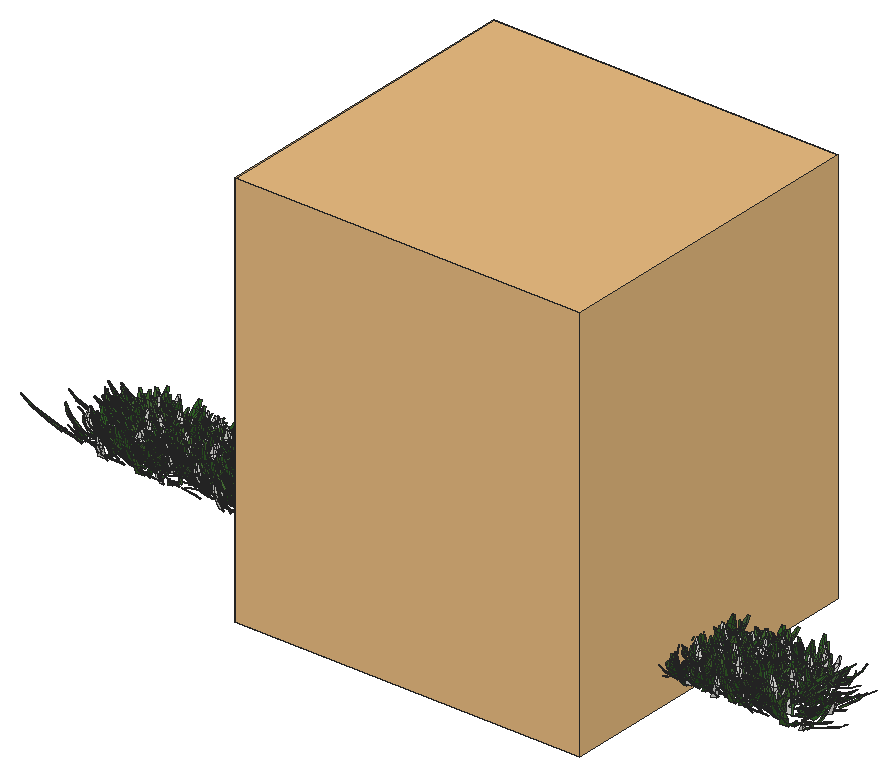
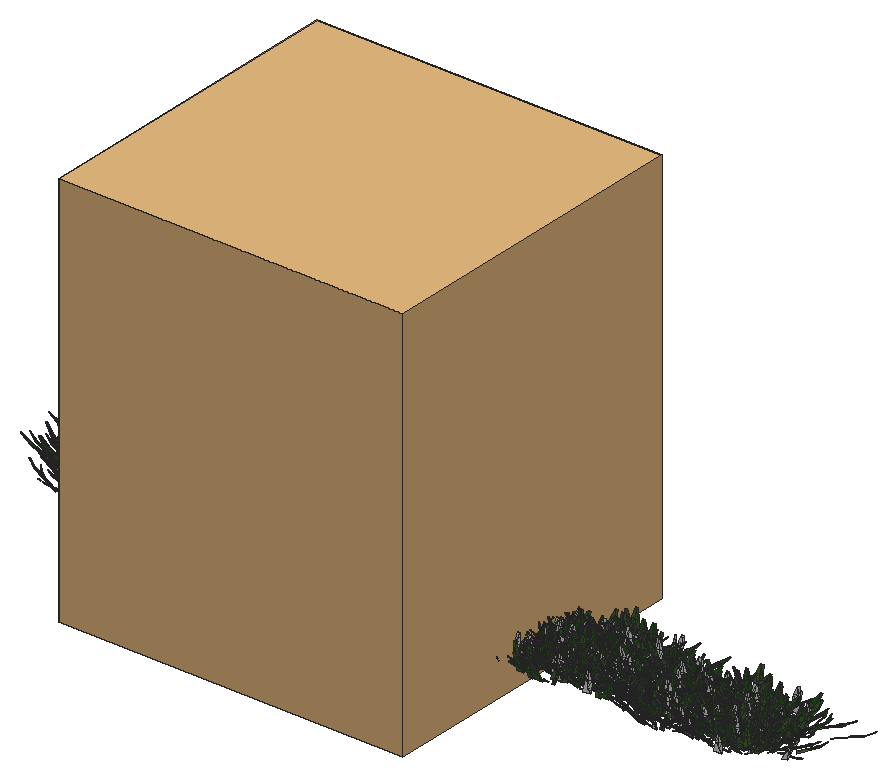
# SketchUp Ruby script. Lengths in inches.
U = 1.inch
M = Sketchup.active_model
def pt(a) = Geom::Point3d.new(a.map { |v| v * U })
def face(e, loops, mat)
  f = e.add_face(loops[0].map { |a| pt(a) })
  loops[1..].each { |l| e.add_face(l.map { |a| pt(a) }).erase! }
  f.material = f.back_material = mat if mat
  f
end
# faces: each face lists its corners as indices into pts; further lists are holes
def faces(e, pts, list, mat = nil) = list.each { |f| face(e, (f[0].is_a?(Array) ? f : [f]).map { |l| l.map { |i| pts[i] } }, mat) }
# xy, xz, yz: faces in a plane at the given z, y or x. An outline is a flat list of corners, or four numbers for a rectangle; further outlines are holes
def ring(l) = l.size == 4 ? [[l[0], l[1]], [l[2], l[1]], [l[2], l[3]], [l[0], l[3]]] : l.each_slice(2).to_a
def flat(e, list, mat, &to3) = list.each { |f| face(e, (f[0].is_a?(Array) ? f : [f]).map { |l| ring(l).map { |u, v| to3.(u, v) } }, mat) }
def xy(e, z, list, mat = nil) = flat(e, list, mat) { |x, y| [x, y, z] }
def xz(e, y, list, mat = nil) = flat(e, list, mat) { |x, z| [x, y, z] }
def yz(e, x, list, mat = nil) = flat(e, list, mat) { |y, z| [x, y, z] }
def lines(e, pts, list) = list.each { |a, b| e.add_line(pt(pts[a]), pt(pts[b])) }
# prism: a flat outline (further loops are holes) pulled along v
def prism(e, loops, v, mat = nil)
  f = face(e, loops, mat); d = Geom::Vector3d.new(v.map { |x| x * U })
  f.pushpull(f.normal.samedirection?(d) ? d.length : -d.length)
end
def box(e, o, s, mat = nil) = prism(e, [[o, [o[0] + s[0], o[1], o[2]], [o[0] + s[0], o[1] + s[1], o[2]], [o[0], o[1] + s[1], o[2]]]], [0, 0, s[2]], mat)
def at(x, y, z, deg = 0) = Geom::Transformation.translation(pt([x, y, z])) * Geom::Transformation.rotation(ORIGIN, Z_AXIS, deg.degrees)
def axes(o, x, y, z) = Geom::Transformation.new([*x, 0, *y, 0, *z, 0, *pt(o).to_a, 1])
def part(name) = M.definitions.add(name)
# library, detail: a bought-in or finely detailed component or shape, given as its bounding box
def library(name, o, s) = part(name).tap { |d| box(d.entities, o, s) }
def detail(e, o, s) = box(e.add_group.entities, o, s)
def put(e, d, t, mat = nil) = e.add_instance(d, t).tap { |i| i.material = mat if mat }
def group(e, t, mat = nil) = e.add_group.tap { |g| g.transformation = t; g.material = mat if mat }.entities
root = M.entities
M.materials.add("Material82").color = [68, 110, 58]
M.materials.add("Material83").color = [48, 90, 38]
M.materials.add("Material84").color = [68, 110, 48]
M.materials.add("Material85").color = [48, 90, 48]
M.materials.add("Material86").color = [58, 110, 58]
M.materials.add("Material87").color = [58, 90, 38]
M.materials.add("Material88").color = [68, 100, 58]
M.materials.add("Material89").color = [48, 100, 38]
c1 = part("grass00")
p = [[-0.6875,0.15,0],[-0.56,0.08,5.52],[-0.04,0.03,2.76],[0.48,-0.02,0],[0.35,-0.02,5.52],[-0.1,-0.14,5.52],
  [-0.12,0.65,8.37],[-0.42,0.65,8.37]]
faces(c1.entities,p,[[0,1,2,3],[3,2,4],[1,5,2],[5,4,2],[1,6,5],[4,5,6],[7,6,1]])
c2 = part("Group16\#1")
put(c2.entities,c1,axes([1.44,-0.61,-0.01],[0.05352,0.12609,0],[-0.10704,0.04543,0.07239],[0.06664,-0.02828,0.11628]),"Material85")
put(c2.entities,c1,axes([0.76,-0.15,-0.01],[0.04676,0.24062,0],[-0.23162,0.04501,0.06642],[0.0652,-0.01267,0.23595]),"Material82")
put(c2.entities,c1,axes([0.79,0.01,-0.01],[-0.00606,0.34651,0],[-0.34381,-0.00602,0.0432],[0.04319,0.00076,0.34386]))
put(c2.entities,c1,axes([1,0.23,-0.01],[-0.07192,0.31144,0],[-0.28722,-0.06632,0.1236],[0.12043,0.02781,0.29478]),"Material84")
put(c2.entities,c1,axes([1.66,0.77,-0.01],[-0.13828,0.29651,0],[-0.21551,-0.1005,0.22471],[0.20365,0.09498,0.23779]),"Material89")
put(c2.entities,c1,axes([0.6875,0.52,-0.01],[-0.18126,0.24051,0],[-0.22746,-0.17142,0.09788],[0.07817,0.05891,0.28481]),"Material84")
put(c2.entities,c1,axes([0.68,0.78,-0.01],[-0.215,0.18688,0],[-0.12385,-0.14248,0.21334],[0.13995,0.16101,0.18878]),"Material82")
put(c2.entities,c1,axes([0.56,1,-0.01],[-0.13756,0.07624,0],[-0.06159,-0.11112,0.0927],[0.04494,0.08108,0.12705]),"Material84")
put(c2.entities,c1,axes([0.2,0.64,-0.01],[-0.23729,0.07254,0],[-0.05711,-0.18681,0.153],[0.04473,0.14632,0.19535]),"Material89")
put(c2.entities,c1,axes([0.0625,0.72,-0.01],[-0.28874,0.02525,0],[-0.02179,-0.24916,0.14647],[0.01276,0.14591,0.25012]),"Material82")
put(c2.entities,c1,axes([-0.08,0.62,-0.01],[-0.34089,-0.04187,0],[0.03255,-0.26504,0.216],[-0.02633,0.21439,0.26703]),"Material89")
put(c2.entities,c1,axes([-0.34,0.98,-0.01],[-0.14314,-0.0493,0],[0.04397,-0.12769,0.06843],[-0.02228,0.0647,0.13505]),"Material89")
put(c2.entities,c1,axes([-0.87,1.45,-0.01],[-0.23488,-0.14114,0],[0.13761,-0.22901,0.06087],[-0.03135,0.05217,0.26717]))
put(c2.entities,c1,axes([-0.72,0.77,-0.01],[-0.14208,-0.13251,0],[0.07209,-0.0773,0.16301],[-0.11118,0.11922,0.1057]),"Material89")
put(c2.entities,c1,axes([-0.62,0.43,-0.01],[-0.14845,-0.21203,0],[0.18654,-0.13061,0.12304],[-0.10079,0.07057,0.22772]),"Material82")
put(c2.entities,c1,axes([-0.68,0.29,-0.01],[-0.13639,-0.32136,0],[0.31723,-0.13464,0.05579],[-0.05136,0.0218,0.34462]),"Material83")
put(c2.entities,c1,axes([-0.64,0.125,-0.01],[-0.0458,-0.23569,0],[0.22124,-0.043,0.08276],[-0.08124,0.01579,0.22538]),"Material86")
put(c2.entities,c1,axes([-1.6,-0.03,-0.01],[0.00576,-0.32897,0],[0.27526,0.00482,0.18018],[-0.18015,-0.00315,0.2753]),"Material84")
put(c2.entities,c1,axes([-1.36,-0.31,-0.01],[0.05718,-0.24765,0],[0.18172,0.04196,0.17267],[-0.16825,-0.03885,0.1865]),"Material89")
put(c2.entities,c1,axes([-1.54,-0.72,-0.01],[0.06537,-0.14017,0],[0.13555,0.06321,0.03939],[-0.0357,-0.01665,0.14956]))
put(c2.entities,c1,axes([-1.19,-0.9,-0.01],[0.09597,-0.12735,0],[0.11214,0.08451,0.07557],[-0.06035,-0.04548,0.14042]),"Material88")
put(c2.entities,c1,axes([-0.47,-0.54,-0.01],[0.11588,-0.10072,0],[0.0618,0.0711,0.12124],[-0.07953,-0.0915,0.0942]))
put(c2.entities,c1,axes([-0.47,-0.84,-0.01],[0.11927,-0.0661,0],[0.06603,0.11913,0.00646],[-0.00313,-0.00565,0.13621]),"Material84")
put(c2.entities,c1,axes([-0.38,-1.24,-0.01],[0.28037,-0.08571,0],[0.0618,0.20215,0.20315],[-0.05939,-0.19428,0.21139]),"Material88")
put(c2.entities,c1,axes([-0.06,-0.66,-0.01],[0.22719,-0.01987,0],[0.01247,0.14255,0.17758],[-0.01547,-0.17691,0.1431]),"Material87")
put(c2.entities,c1,axes([0.11,-0.89,-0.01],[0.14882,0.01828,0],[-0.01058,0.08611,0.12229],[0.01491,-0.12138,0.08676]),"Material85")
put(c2.entities,c1,axes([0.25,-0.72,-0.01],[0.20481,0.07053,0],[-0.06206,0.18022,0.10291],[0.03351,-0.0973,0.1906]),"Material85")
put(c2.entities,c1,axes([0.85,-1.42,-0.01],[0.16481,0.09904,0],[-0.09472,0.15762,0.05616],[0.02893,-0.04814,0.18389]),"Material84")
put(c2.entities,c1,axes([1.01,-1.09,-0.01],[0.21858,0.20385,0],[-0.17495,0.1876,0.15339],[0.10462,-0.11218,0.25652]),"Material89")
put(c2.entities,c1,axes([1.01,-0.71,-0.01],[0.08733,0.12473,0],[-0.06445,0.04512,0.13037],[0.1068,-0.07477,0.07867]),"Material85")
c3 = part("Group15\#1")
put(c3.entities,c2,at(0,0,0))
c4 = part("3darcstudiotree_grass00\#1")
put(c4.entities,c3,at(0,0,0))
c5 = library("Flora+17",[-57.52,158.6,-38.64],[66.99,62.88,77.28])
put(root,c4,axes([1787.23,367.59,-34.17],[-1.07809,1.72568,0],[-4.31745,-0.4195,-0.00818],[-0.04348,-0.00422,1.82396]))
put(root,c4,axes([1792.84,368.1,-34.17],[4.00543,0.63259,0],[-1.51384,1.49079,-0.05201],[-0.11143,0.10973,1.75905]))
put(root,c4,axes([1834.72,368.38,-34.17],[-2.53432,-1.16731,0],[3.13366,-1.05813,-0.03189],[0.12006,-0.04054,1.53238]))
put(root,c4,axes([1804.73,368.98,-34.17],[2.98326,-0.56932,0],[1.56375,1.27443,-0.0104],[0.02417,0.0197,1.43546]))
put(root,c4,axes([1783.02,368.18,-34.17],[-2.79487,1.34009,0],[-3.4856,-1.13062,-0.01702],[-0.07434,-0.02411,1.91367]))
put(root,c4,axes([1843.875,368.37,-34.17],[-1.68076,1.66641,0],[-3.14491,-0.49334,-0.04072],[-0.22908,-0.03594,1.53595]))
put(root,c4,axes([1820.36,368.59,-34.17],[0.66214,1.69294,0],[-3.60919,0.21955,-0.0058],[-0.03794,0.00231,1.813]))
put(root,c4,axes([1870.35,368.72,-34.17],[-3.64575,-0.40954,0],[1.09452,-1.51542,-0.03955],[0.07063,-0.09779,1.95202]))
put(root,c4,axes([1779.59,368.83,-34.17],[-3.63168,-0.94551,0],[2.04917,-1.22414,-0.0411],[0.11661,-0.06966,1.43569]))
put(root,c4,axes([1860.89,368.6875,-34.17],[-4.50339,0.12702,0],[-0.32923,-1.8154,-0.06114],[-0.02191,-0.12082,1.73764]))
put(root,c4,axes([1875.55,369.12,-34.17],[3.9368,0.32867,0],[-0.7645,1.42421,-0.03259],[-0.03941,0.07343,1.61556]))
put(root,c4,axes([1848.03,369.1,-34.17],[-1.97756,-1.20873,0],[2.87461,-0.73146,-0.04434],[0.19177,-0.0488,1.31982]))
put(root,c4,axes([1817.45,368.64,-34.17],[-0.80195,1.7338,0],[-4.65742,-0.33505,-0.02378],[-0.12913,-0.00929,1.95907]))
put(root,c4,axes([1767.8,368.9375,-34.17],[1.69594,1.55136,0],[-4.25972,0.72425,-0.01792],[-0.06344,0.01079,1.34035]))
put(root,c4,axes([1887.4,368.75,-34.17],[-0.96856,1.32293,0],[-4.17213,-0.47507,-0.01983],[-0.0846,-0.00963,1.44555]))
put(root,c4,axes([1865.01,368.93,-34.17],[-4.11343,-0.37841,0],[0.77008,-1.30194,-0.01564],[0.01915,-0.03238,1.3694]))
put(root,c4,axes([1762.23,368.84,-34.17],[-1.08101,1.66314,0],[-4.29936,-0.43462,-0.05431],[-0.26643,-0.02693,1.6847]))
put(root,c4,axes([1779.23,369.72,-34.17],[3.51633,-0.36112,0],[0.9428,1.4278,-0.03218],[0.03818,0.05783,1.32043]))
put(root,c4,axes([1809.87,369,-34.17],[-3.19418,0.83767,0],[-2.09756,-1.24397,-0.00165],[-0.00457,-0.00271,1.42237]))
put(root,c4,axes([1817.79,369.79,-34.17],[4.46941,0.03034,0],[-0.07094,1.62545,-0.04862],[-0.00377,0.08633,1.39123]))
put(root,c4,axes([1840.21,370.15,-34.17],[3.30112,0.44872,0],[-1.07202,1.22659,-0.01199],[-0.02088,0.02389,1.31812]))
put(root,c4,axes([1831.125,369.98,-34.17],[2.54447,1.0037,0],[-2.66541,1.05092,-0.04694],[-0.19938,0.07861,1.69685]))
put(root,c4,axes([1796.16,369.8,-34.17],[-2.46131,1.0799,0],[-2.93079,-1.03891,-0.05045],[-0.18868,-0.06689,1.48531]))
put(root,c4,axes([1844.53,370.08,-34.17],[1.71949,1.25443,0],[-3.5766,0.76249,-0.00296],[-0.01327,0.00283,1.55057]))
put(root,c4,axes([1754.76,369.73,-34.17],[-4.32286,0.64319,0],[-1.64772,-1.72238,-0.03096],[-0.05617,-0.05872,1.79846]))
put(root,c4,axes([1876.98,369.84,-34.17],[-0.85979,1.68043,0],[-3.51636,-0.27982,-0.00527],[-0.03686,-0.00293,1.91768]))
put(root,c4,axes([1788.52,370.32,-34.17],[-1.06768,-1.28552,0],[4.42505,-0.5716,-0.01545],[0.0652,-0.00842,1.54954]))
put(root,c4,axes([1804.84,370.78,-34.17],[1.44921,-1.37247,0],[3.47001,0.56986,-0.04485],[0.23379,0.03839,1.59096]))
put(root,c4,axes([1851.11,371.03,-34.17],[2.98286,-1.36319,0],[2.94856,1.00345,-0.04774],[0.23651,0.08049,1.91023]))
put(root,c4,axes([1829.28,370.375,-34.17],[-4.5512,0.12899,0],[-0.29843,-1.6376,-0.01837],[-0.00647,-0.03552,1.53349]))
put(root,c4,axes([1762.11,370.79,-34.17],[2.63123,0.92373,0],[-2.85346,1.26414,-0.03405],[-0.11674,0.05172,1.65877]))
put(root,c4,axes([1881.76,371.19,-34.17],[2.31859,-1.24057,0],[3.7429,1.08799,-0.00987],[0.04342,0.01262,1.9048]))
put(root,c4,axes([1854.8,370.77,-34.17],[3.00883,1.26771,0],[-3.0504,1.12602,-0.05678],[-0.17699,0.06533,1.337]))
put(root,c4,axes([1867.03,371.19,-34.17],[2.02967,-1.41693,0],[3.62772,0.8082,-0.05349],[0.29346,0.06538,1.96798]))
put(root,c4,axes([1812.2,371.26,-34.17],[3.59827,-1.20315,0],[2.55541,1.18863,-0.04452],[0.1901,0.08842,1.95574]))
put(root,c4,axes([1820.14,370.5,-34.17],[-2.59269,1.36416,0],[-3.43206,-1.0145,-0.01976],[-0.08545,-0.02526,1.7373]))
put(root,c4,axes([1797.97,370.72,-34.17],[0.38941,1.44392,0],[-4.06327,0.17043,-0.05804],[-0.26328,0.01104,1.39706]))
put(root,c4,axes([1784.7,371.14,-34.17],[-0.85342,-1.31702,0],[3.52172,-0.35493,-0.03508],[0.23842,-0.02403,1.91126]))
put(root,c4,axes([1872.35,371.09,-34.17],[-1.26608,-1.23533,0],[3.94424,-0.62872,-0.05241],[0.25484,-0.04062,1.67241]))
put(root,c4,axes([1767.44,371.22,-34.17],[2.49471,1.02577,0],[-2.71621,1.02741,-0.02632],[-0.13149,0.04974,1.95302]))
put(root,c4,axes([1860.57,371.13,-34.17],[-2.51394,1.47726,0],[-3.35133,-0.88701,-0.03945],[-0.17377,-0.04599,1.6047]))
put(root,c4,axes([1772.59,371.15,-34.17],[-3.75575,0.69708,0],[-1.71963,-1.441,-0.0027],[-0.006,-0.00502,1.57765]))
put(root,c4,axes([1815.45,372.17,-34.17],[4.01141,-0.57098,0],[1.38004,1.50792,-0.00463],[0.00922,0.01007,1.7876]))
put(root,c4,axes([1831.35,372.35,-34.17],[1.0408,-1.70786,0],[3.59221,0.34047,-0.00397],[0.02558,0.00242,1.83602]))
put(root,c4,axes([1883.92,371.99,-34.17],[1.31466,1.33352,0],[-4.27103,0.65487,-0.01993],[-0.10773,0.01652,1.99239]))
put(root,c4,axes([1819.9,372.54,-34.17],[4.23995,-0.14734,0],[0.39715,1.77755,-0.00682],[0.00263,0.01179,1.49182]))
put(root,c4,axes([1803.74,371.97,-34.17],[-3.94041,-0.17555,0],[0.52244,-1.82386,-0.03054],[0.01805,-0.06303,1.83699]))
put(root,c4,axes([1766.88,372,-34.17],[-3.80907,0.85988,0],[-1.7501,-1.20575,-0.03218],[-0.10036,-0.06914,1.65786]))
put(root,c4,axes([1878.52,372.31,-34.17],[3.99583,0.96728,0],[-1.88023,1.20803,-0.0354],[-0.13352,0.08578,1.94218]))
put(root,c4,axes([1850.35,372.2,-34.17],[1.07934,1.49635,0],[-4.41478,0.49528,-0.01266],[-0.0607,0.00681,1.71446]))
put(root,c4,axes([1795.8,372.04,-34.17],[-1.53161,1.39817,0],[-3.93212,-0.66992,-0.05011],[-0.24211,-0.04125,1.6899]))
put(root,c4,axes([1759.02,372.73,-34.17],[0.46065,-1.85098,0],[4.3401,0.16799,-0.05803],[0.23131,0.00895,1.30918]))
put(root,c4,axes([1775.79,372.1,-34.17],[-2.75394,0.84395,0],[-2.86283,-1.45294,-0.03993],[-0.13572,-0.06888,1.9372]))
put(root,c4,axes([1838.96,372.39,-34.17],[-3.99444,-0.7583,0],[1.47781,-1.21073,-0.01121],[0.03612,-0.02959,1.89718]))
put(root,c4,axes([1756.58,372.38,-34.17],[-2.97002,-0.61033,0],[1.81963,-1.37718,-0.0201],[0.04091,-0.03096,1.30027]))
put(root,c4,axes([1870.91,372.29,-34.17],[0.15484,1.66312,0],[-4.06716,0.05889,-0.05084],[-0.28361,0.00411,1.70302]))
put(root,c4,axes([1810.59,372.22,-34.17],[-1.75851,1.2095,0],[-3.69968,-0.83659,-0.01882],[-0.09945,-0.02249,1.94745]))
put(root,c4,axes([1856.28,372.6875,-34.17],[1.72171,1.1824,0],[-3.73214,0.84521,-0.0451],[-0.23455,0.05312,1.93445]))
put(root,c4,axes([1867.02,373.33,-34.17],[0.19619,-1.71635,0],[3.31321,0.0589,-0.03915],[0.30696,0.00546,1.95085]))
put(root,c4,axes([1801.13,372.79,-34.17],[-0.47592,1.56401,0],[-3.26389,-0.15447,-0.01529],[-0.10295,-0.00487,1.67142]))
put(root,c4,axes([1773.59,372.97,-34.17],[-0.69376,1.57067,0],[-3.29157,-0.22612,-0.03897],[-0.27242,-0.01871,1.77692]))
put(root,c4,axes([1786.71,372.93,-34.17],[-3.02696,1.26281,0],[-2.89442,-1.07905,-0.01805],[-0.07526,-0.02806,1.71251]))
put(root,c4,axes([1844.62,373.11,-34.17],[-0.66988,1.5554,0],[-4.19746,-0.28116,-0.06003],[-0.34231,-0.02293,1.84592]))
put(root,c4,axes([1784.48,373.2,-34.17],[-1.89755,1.14164,0],[-2.79539,-0.72263,-0.04],[-0.1948,-0.05036,1.45882]))
put(root,c4,axes([1828.21,373.36,-34.17],[-1.94069,1.13311,0],[-3.87728,-1.03282,-0.01862],[-0.08293,-0.02209,1.88514]))
put(root,c4,axes([1856.08,374.12,-34.17],[1.1935,-1.34336,0],[4.3339,0.59885,-0.02001],[0.09738,0.01346,1.77455]))
put(root,c4,axes([1859.83,373.36,-34.17],[-2.50228,1.03927,0],[-3.36492,-1.26006,-0.01749],[-0.0653,-0.02445,1.7911]))
put(root,c4,axes([1756.82,374.14,-34.17],[3.05945,-1.08948,0],[2.66485,1.16389,-0.04418],[0.16678,0.07284,1.67893]))
put(root,c4,axes([1782.98,374.46,-34.17],[4.28763,0.74332,0],[-1.60811,1.44267,-0.02572],[-0.05083,0.0456,1.47108]))
put(root,c4,axes([1869.86,374.74,-34.17],[3.2454,-0.59836,0],[1.90263,1.60498,-0.04906],[0.1129,0.09524,1.82977]))
put(root,c4,axes([1798.79,374.5,-34.17],[-3.62624,-0.35306,0],[1.02554,-1.63824,-0.03453],[0.0374,-0.05975,1.44935]))
put(root,c4,axes([1788.71,374.81,-34.17],[4.10391,0.70985,0],[-1.57565,1.41679,-0.04488],[-0.12117,0.10895,1.97665]))
put(root,c4,axes([1821.97,374.5,-34.17],[-4.00947,-0.30727,0],[0.87061,-1.76683,-0.00093],[0.00074,-0.0015,1.42207]))
put(root,c4,axes([1851.14,375.04,-34.17],[3.36205,-0.0702,0],[0.18049,1.34442,-0.02933],[0.01197,0.08919,1.97542]))
put(root,c4,axes([1886.81,374.89,-34.17],[-3.24576,-0.77305,0],[1.70346,-1.11239,-0.04514],[0.15554,-0.10157,1.64638]))
put(root,c4,axes([1859.58,374.53,-34.17],[-2.83529,0.94791,0],[-2.49489,-1.16063,-0.0209],[-0.0692,-0.03219,1.48072]))
put(root,c4,axes([1816.33,375.3,-34.17],[2.86215,-0.69885,0],[2.15737,1.37418,-0.03178],[0.09016,0.05743,1.65559]))
put(root,c4,axes([1866.41,374.86,-34.17],[-4.36996,-0.43983,0],[0.81337,-1.25688,-0.00096],[0.00152,-0.00235,1.58162]))
put(root,c4,axes([1792.21,375.43,-34.17],[3.05285,-0.84724,0],[2.57962,1.44566,-0.04926],[0.16288,0.09128,1.93034]))
put(root,c4,axes([1830.85,375,-34.17],[2.0306,1.51402,0],[-3.86929,0.80712,-0.01033],[-0.04249,0.00886,1.52631]))
put(root,c4,axes([1775.57,374.91,-34.17],[-4.22095,0.29279,0],[-0.61258,-1.3735,-0.03096],[-0.02808,-0.06297,1.38775]))
put(root,c4,axes([1772.56,375.08,-34.17],[-3.27374,-0.87824,0],[2.36689,-1.37221,-0.01911],[0.04526,-0.02624,1.32815]))
put(root,c4,axes([1764.81,375.66,-34.17],[1.2731,-1.20941,0],[3.44603,0.56418,-0.03248],[0.17294,0.02831,1.61223]))
put(root,c4,axes([1811.41,375.47,-34.17],[2.55345,1.05656,0],[-3.3838,1.27189,-0.0237],[-0.06613,0.02486,1.35093]))
put(root,c4,axes([1759,375.25,-34.17],[1.1355,1.36945,0],[-3.88951,0.50159,-0.05705],[-0.27012,0.03483,1.52794]))
put(root,c4,axes([1840.08,375.57,-34.17],[4.32541,0.68003,0],[-1.26335,1.24977,-0.02018],[-0.04043,0.04,1.38364]))
put(root,c4,axes([1806.65,375.13,-34.17],[-2.26024,1.36544,0],[-3.77789,-0.97262,-0.02867],[-0.12669,-0.03262,1.78429]))
put(root,c4,axes([1877.2,375.37,-34.17],[-1.11192,1.29739,0],[-3.39488,-0.45252,-0.04196],[-0.24016,-0.03201,1.62262]))
put(root,c4,axes([1844.73,375.57,-34.17],[-3.14118,-0.50543,0],[1.51948,-1.46871,-0.03312],[0.08056,-0.07787,1.94116]))
put(root,c4,axes([1884.03,375.41,-34.17],[-3.94382,0.34286,0],[-0.79478,-1.42188,-0.01188],[-0.01845,-0.03301,1.99665]))
put(root,c4,axes([1828.69,375.51,-34.17],[-4.08544,0.78173,0],[-2.02978,-1.64985,-0.06144],[-0.10479,-0.08517,1.3618]))
put(root,c4,axes([1866.21,376.3,-34.17],[0.47621,-1.80202,0],[3.38439,0.1391,-0.02929],[0.17813,0.00732,1.55926]))
put(root,c4,axes([1784.18,376.72,-34.17],[3.68176,-0.08889,0],[0.28452,1.83295,-0.0507],[0.01477,0.09515,1.66388]))
put(root,c4,axes([1881.39,376.84,-34.17],[4.51376,-0.38644,0],[0.93116,1.69158,-0.03342],[0.04124,0.07493,1.91382]))
put(root,c4,axes([1779.45,376.99,-34.17],[3.55776,-0.23199,0],[0.75341,1.79699,-0.01648],[0.0118,0.02815,1.51991]))
put(root,c4,axes([1787.02,376.23,-34.17],[-2.26269,0.97698,0],[-3.46591,-1.24844,-0.00484],[-0.01583,-0.0057,1.55938]))
put(root,c4,axes([1772.44,376.53,-34.17],[-0.84248,1.5623,0],[-4.12413,-0.34589,-0.02719],[-0.15102,-0.01267,1.79436]))
put(root,c4,axes([1814.4,376.78,-34.17],[1.45585,1.40356,0],[-4.29762,0.69331,-0.06498],[-0.33385,0.05386,1.93183]))
put(root,c4,axes([1820.1,377.44,-34.17],[2.50638,-0.90958,0],[2.96207,1.26944,-0.00074],[0.00258,0.00111,1.68668]))
put(root,c4,axes([1849.2,377.34,-34.17],[2.93855,-0.93601,0],[2.3882,1.16609,-0.03491],[0.14245,0.06955,1.84986]))
put(root,c4,axes([1837.01,377.17,-34.17],[3.70843,0.7821,0],[-1.67561,1.2357,-0.00407],[-0.01146,0.00845,1.59208]))
put(root,c4,axes([1759.82,377.26,-34.17],[-2.75759,-1.29294,0],[3.16062,-1.04842,-0.04595],[0.19898,-0.066,1.75181]))
put(root,c4,axes([1859.14,377.08,-34.17],[-3.51736,-0.62046,0],[1.43276,-1.26324,-0.00732],[0.0191,-0.01684,1.68082]))
put(root,c5,at(1856.24,187.19,0))
put(root,c4,axes([1875.51,377.58,-34.17],[1.17526,-1.64902,0],[4.03097,0.44682,-0.04021],[0.21409,0.02373,1.73573]))
put(root,c4,axes([1754.09,377.43,-34.17],[3.8564,0.72862,0],[-1.8534,1.52567,-0.04599],[-0.08438,0.06946,1.36526]))
put(root,c4,axes([1806.79,377.73,-34.17],[2.63553,-1.14097,0],[3.49929,1.25715,-0.04921],[0.17097,0.06142,1.66765]))
put(root,c4,axes([1827.25,377.46,-34.17],[-2.13357,-1.0721,0],[3.45076,-1.06807,-0.04646],[0.2021,-0.06255,1.81816]))
put(root,c4,axes([1873.25,377.69,-34.17],[3.33693,-0.09981,0],[0.31842,1.6558,-0.06006],[0.02203,0.11454,1.53056]))
put(root,c4,axes([1843.68,377.86,-34.17],[1.17971,-1.62892,0],[3.63954,0.40996,-0.01145],[0.05532,0.00623,1.42532]))
put(root,c4,axes([1792.52,377.29,-34.17],[-4.27172,-0.34301,0],[0.88739,-1.71879,-0.03896],[0.04123,-0.07985,1.76791]))
put(root,c4,axes([1812.66,377.48,-34.17],[1.4209,1.26091,0],[-3.92098,0.6872,-0.00487],[-0.02309,0.00405,1.66894]))
put(root,c4,axes([1853.99,377.52,-34.17],[-2.4369,-0.91248,0],[2.76412,-1.14811,-0.01822],[0.07791,-0.03236,1.86907]))
put(root,c4,axes([1799.59,377.49,-34.17],[-4.07234,0.0884,0],[-0.21728,-1.55677,-0.00024],[-0.00008,-0.0006,1.85086]))
put(root,c4,axes([1764.37,377.59,-34.17],[-0.67685,1.82709,0],[-3.63349,-0.20935,-0.03578],[-0.17247,-0.00994,1.34076]))
put(root,c4,axes([1831.9,377.67,-34.17],[-4.28311,0.42951,0],[-0.86146,-1.33607,-0.01716],[-0.03026,-0.04692,1.87475]))
put(root,c4,axes([1834.18,378.42,-34.17],[3.93391,0.38635,0],[-0.92741,1.4687,-0.04825],[-0.05916,0.09369,1.45973]))
put(root,c4,axes([1845.93,378.82,-34.17],[1.5424,-1.39232,0],[4.02917,0.6942,-0.02716],[0.11079,0.01909,1.46706]))
put(root,c4,axes([1854.64,378.64,-34.17],[-3.14575,-1.33265,0],[2.56413,-0.94137,-0.04944],[0.22162,-0.08136,1.60821]))
put(root,c4,axes([1871.36,378.89,-34.17],[3.16271,-0.89527,0],[1.91794,1.05379,-0.02763],[0.08663,0.0476,1.3256]))
put(root,c4,axes([1767.79,378.85,-34.17],[4.09109,-0.59758,0],[1.20224,1.2801,-0.03178],[0.07676,0.08173,1.80429]))
put(root,c4,axes([1817.58,378.84,-34.17],[0.03648,-1.32003,0],[3.51668,0.01511,-0.01263],[0.08154,0.00035,1.70174]))
put(root,c4,axes([1836.73,378.8,-34.17],[2.84603,0.80034,0],[-2.3016,1.27293,-0.03635],[-0.10022,0.05543,1.41103]))
put(root,c4,axes([1823.4375,379.15,-34.17],[0.45602,-1.75469,0],[4.51141,0.18235,-0.06373],[0.28019,0.01133,1.50237]))
put(root,c4,axes([1862.21,378.88,-34.17],[2.37182,1.09167,0],[-3.5393,1.19596,-0.05975],[-0.18065,0.06104,1.3909]))
put(root,c4,axes([1793.56,379.19,-34.17],[4.21739,-0.2744,0],[0.59088,1.41243,-0.03976],[0.04192,0.1002,1.7619]))
put(root,c4,axes([1776.67,378.73,-34.17],[-4.11616,0.08361,0],[-0.21641,-1.65704,-0.00589],[-0.00131,-0.01,1.35922]))
put(root,c4,axes([1755,379,-34.17],[1.39303,1.55232,0],[-3.39855,0.47433,-0.0171],[-0.11021,0.01538,1.84743]))
put(root,c4,axes([1866.02,379.62,-34.17],[1.48234,-1.44208,0],[4.35208,0.69577,-0.03495],[0.16928,0.02706,1.83937]))
put(root,c4,axes([1827.82,378.91,-34.17],[-3.86986,1.0079,0],[-2.20275,-1.31539,-0.01955],[-0.05283,-0.03155,1.46911]))
put(root,c4,axes([1881.65,379.78,-34.17],[2.23867,-1.3669,0],[3.69886,0.94218,-0.0579],[0.27243,0.06939,1.84885]))
put(root,c4,axes([1877.71,379.52,-34.17],[-1.90503,-1.23869,0],[3.27066,-0.78232,-0.01057],[0.0584,-0.01397,1.85267]))
put(root,c4,axes([1759.34,379.89,-34.17],[2.18609,-1.17283,0],[3.5885,1.04029,-0.0227],[0.08817,0.02556,1.60931]))
put(root,c4,axes([1788.18,379.79,-34.17],[4.1241,0.10126,0],[-0.23149,1.46627,-0.04181],[-0.01816,0.11501,1.95138]))
put(root,c4,axes([1803.86,379.4,-34.17],[-3.62534,0.37466,0],[-0.93047,-1.40031,-0.00505],[-0.0081,-0.01218,1.74136]))
put(root,c4,axes([1784.31,379.48,-34.17],[-4.14933,0.35699,0],[-0.86081,-1.55612,-0.03649],[-0.04634,-0.08377,1.80375]))
put(root,c4,axes([1812.125,379.87,-34.17],[-1.44336,-1.26835,0],[3.91991,-0.69378,-0.01184],[0.05292,-0.00937,1.57815]))
put(root,c4,axes([1771.57,379.66,-34.17],[-3.20067,0.8851,0],[-2.09814,-1.18003,-0.04222],[-0.15558,-0.0875,1.75818]))
put(root,c4,axes([1848.34,379.85,-34.17],[-2.84152,0.97731,0],[-2.62045,-1.18497,-0.0546],[-0.22213,-0.10045,1.84968]))
put(root,c4,axes([1797.6875,380,-34.17],[0.82539,1.5958,0],[-3.41483,0.2747,-0.03877],[-0.28197,0.02268,1.93915]))
put(root,c4,axes([1810.15,380.81,-34.17],[4.36048,0.20882,0],[-0.42656,1.38529,-0.01966],[-0.01597,0.05186,1.78732]))
put(root,c4,axes([1760.47,381.05,-34.17],[4.28771,-0.12133,0],[0.32919,1.80935,-0.01186],[0.00375,0.02059,1.52253]))
put(root,c4,axes([1846.01,380.65,-34.17],[-2.28475,-0.97473,0],[2.77585,-1.01196,-0.01026],[0.04604,-0.01678,1.73127]))
put(root,c4,axes([1875.375,380.61,-34.17],[1.07114,1.64692,0],[-4.05863,0.41055,-0.04684],[-0.20509,0.02075,1.41954]))
put(root,c4,axes([1804.125,380.63,-34.17],[0.44153,1.60869,0],[-4.59886,0.19631,-0.03135],[-0.13775,0.00588,1.53244]))
put(root,c4,axes([1839.83,380.7,-34.17],[0.72726,1.40914,0],[-3.71927,0.29854,-0.02796],[-0.18755,0.01505,1.94708]))
put(root,c4,axes([1816.05,380.86,-34.17],[2.07536,1.00802,0],[-2.97078,0.95128,-0.04172],[-0.20153,0.06453,1.78477]))
put(root,c4,axes([1823.1,381.11,-34.17],[-2.23262,-1.3088,0],[3.58665,-0.95157,-0.0439],[0.1738,-0.04611,1.54604]))
put(root,c4,axes([1856.2,381.24,-34.17],[-2.0126,-1.62184,0],[4.11765,-0.79471,-0.06506],[0.29073,-0.05611,1.70958]))
put(root,c4,axes([1848.5,380.65,-34.17],[-3.10197,1.07124,0],[-2.38472,-1.07399,-0.00238],[-0.01101,-0.00496,1.90825]))
put(root,c4,axes([1865.7,380.9,-34.17],[-3.67787,-0.26396,0],[0.66039,-1.43112,-0.02729],[0.03307,-0.07167,1.8715]))
put(root,c4,axes([1872.82,381.46,-34.17],[-0.88129,-1.68738,0],[3.67182,-0.29826,-0.02826],[0.15697,-0.01275,1.59374]))
put(root,c4,axes([1792.5,380.95,-34.17],[-2.93173,0.8474,0],[-2.63832,-1.41962,-0.02359],[-0.06961,-0.03745,1.66971]))
put(root,c4,axes([1770.48,381.68,-34.17],[-0.92548,-1.44714,0],[3.73119,-0.37112,-0.02503],[0.12441,-0.01237,1.47852]))
put(root,c4,axes([1833.38,381.72,-34.17],[-1.15236,-1.67434,0],[3.65122,-0.39084,-0.0298],[0.14551,-0.01558,1.43464]))
put(root,c4,axes([1882.86,381.48,-34.17],[0.85919,1.59494,0],[-3.67668,0.30804,-0.01067],[-0.0678,0.00568,1.82972]))
